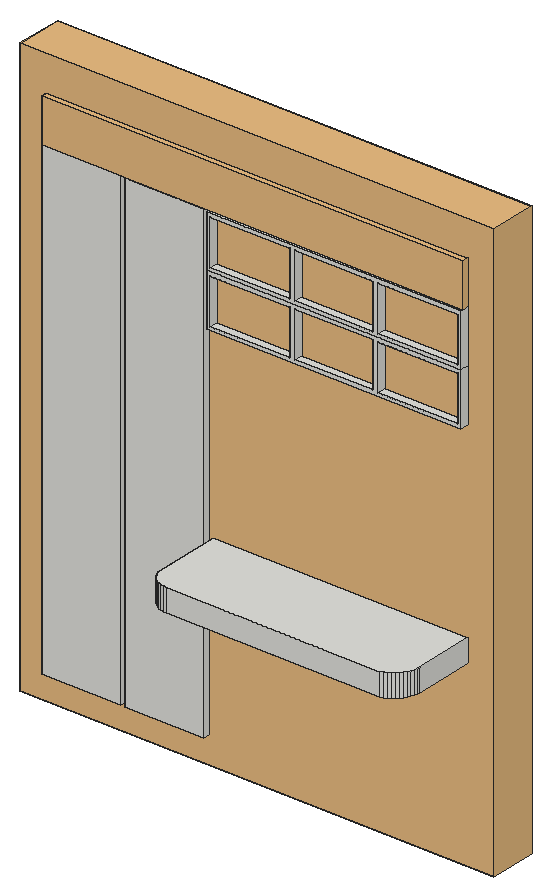
# SketchUp Ruby script. Lengths in inches.
U = 1.inch
M = Sketchup.active_model
def pt(a) = Geom::Point3d.new(a.map { |v| v * U })
def face(e, loops, mat)
  f = e.add_face(loops[0].map { |a| pt(a) })
  loops[1..].each { |l| e.add_face(l.map { |a| pt(a) }).erase! }
  f.material = f.back_material = mat if mat
  f
end
# faces: each face lists its corners as indices into pts; further lists are holes
def faces(e, pts, list, mat = nil) = list.each { |f| face(e, (f[0].is_a?(Array) ? f : [f]).map { |l| l.map { |i| pts[i] } }, mat) }
# xy, xz, yz: faces in a plane at the given z, y or x. An outline is a flat list of corners, or four numbers for a rectangle; further outlines are holes
def ring(l) = l.size == 4 ? [[l[0], l[1]], [l[2], l[1]], [l[2], l[3]], [l[0], l[3]]] : l.each_slice(2).to_a
def flat(e, list, mat, &to3) = list.each { |f| face(e, (f[0].is_a?(Array) ? f : [f]).map { |l| ring(l).map { |u, v| to3.(u, v) } }, mat) }
def xy(e, z, list, mat = nil) = flat(e, list, mat) { |x, y| [x, y, z] }
def xz(e, y, list, mat = nil) = flat(e, list, mat) { |x, z| [x, y, z] }
def yz(e, x, list, mat = nil) = flat(e, list, mat) { |y, z| [x, y, z] }
def lines(e, pts, list) = list.each { |a, b| e.add_line(pt(pts[a]), pt(pts[b])) }
# prism: a flat outline (further loops are holes) pulled along v
def prism(e, loops, v, mat = nil)
  f = face(e, loops, mat); d = Geom::Vector3d.new(v.map { |x| x * U })
  f.pushpull(f.normal.samedirection?(d) ? d.length : -d.length)
end
def box(e, o, s, mat = nil) = prism(e, [[o, [o[0] + s[0], o[1], o[2]], [o[0] + s[0], o[1] + s[1], o[2]], [o[0], o[1] + s[1], o[2]]]], [0, 0, s[2]], mat)
def at(x, y, z, deg = 0) = Geom::Transformation.translation(pt([x, y, z])) * Geom::Transformation.rotation(ORIGIN, Z_AXIS, deg.degrees)
def axes(o, x, y, z) = Geom::Transformation.new([*x, 0, *y, 0, *z, 0, *pt(o).to_a, 1])
def part(name) = M.definitions.add(name)
# library, detail: a bought-in or finely detailed component or shape, given as its bounding box
def library(name, o, s) = part(name).tap { |d| box(d.entities, o, s) }
def detail(e, o, s) = box(e.add_group.entities, o, s)
def put(e, d, t, mat = nil) = e.add_instance(d, t).tap { |i| i.material = mat if mat }
def group(e, t, mat = nil) = e.add_group.tap { |g| g.transformation = t; g.material = mat if mat }.entities
root = M.entities
c1 = library("Group\#5",[0,-12,0],[96,12,10])
xz(root,30,[[44.8,84.8,63,95.2],[64.2,84.8,81.8,95.2],[83,84.8,101.2,95.2]])
detail(root,[0,19.34,-6],[108,10.66,132])
g1 = group(root,at(0,30,-6))
xz(g1,0,[[[0,0,108,132],[5,5,103,127]]])
g2 = group(root,at(44,30,35.4))
xy(g2,0,[[4.82,-30,4.13,-29.95,3.45,-29.8,2.79,-29.56,2.18,-29.22,1.62,-28.8,1.13,-28.31,0.71,-27.75,0.38,-27.13,0.14,-26.48,0,-25.83,0,1.0625,58,1.0625,58,-24.4375,57.96,-24.89,57.82,-25.59,57.6,-26.27,57.3,-26.93,56.92,-27.54,56.48,-28.11,55.98,-28.62,55.42,-29.07,54.81,-29.46,54.16,-29.77,53.48,-30]])
xy(g2,5.2,[[4.82,-30,53.48,-30,54.16,-29.77,54.81,-29.46,55.42,-29.07,55.98,-28.62,56.48,-28.11,56.92,-27.54,57.3,-26.93,57.6,-26.27,57.82,-25.59,57.96,-24.89,58,-24.4375,58,1.0625,0,1.0625,0,-25.83,0.14,-26.48,0.38,-27.13,0.71,-27.75,1.13,-28.31,1.62,-28.8,2.18,-29.22,2.79,-29.56,3.45,-29.8,4.13,-29.95],[58,-24.4375,58.02,-24.17,58,-23.45]])
xz(g2,-30,[[4.82,0,53.48,5.2]])
xz(g2,1.0625,[[0,0,58,5.2]])
yz(g2,0,[[-25.83,0,1.0625,5.2]])
yz(g2,58,[[-24.4375,0,1.0625,5.2]])
p = [[4.13,-29.95,5.2],[3.45,-29.8,5.2],[3.45,-29.8,0],[4.13,-29.95,0],[4.82,-30,5.2],[4.82,-30,0],
  [54.16,-29.77,5.2],[53.48,-30,5.2],[53.48,-30,0],[54.16,-29.77,0],[2.79,-29.56,5.2],[2.79,-29.56,0],
  [54.81,-29.46,5.2],[54.81,-29.46,0],[2.18,-29.22,5.2],[2.18,-29.22,0],[55.42,-29.07,5.2],[55.42,-29.07,0],
  [1.62,-28.8,5.2],[1.62,-28.8,0],[55.98,-28.62,5.2],[55.98,-28.62,0],[1.13,-28.31,5.2],[1.13,-28.31,0],
  [56.48,-28.11,5.2],[56.48,-28.11,0],[0.71,-27.75,5.2],[0.71,-27.75,0],[56.92,-27.54,5.2],[56.92,-27.54,0],
  [0.38,-27.13,5.2],[0.38,-27.13,0],[57.3,-26.93,5.2],[57.3,-26.93,0],[0.14,-26.48,5.2],[0.14,-26.48,0],
  [57.6,-26.27,5.2],[57.6,-26.27,0],[0,-25.83,5.2],[0,-25.83,0],[57.82,-25.59,5.2],[57.82,-25.59,0],
  [57.96,-24.89,5.2],[57.96,-24.89,0],[58,-24.4375,5.2],[58,-24.4375,0]]
faces(g2,p,[[0,1,2,3],[4,0,3,5],[6,7,8,9],[1,10,11,2],[12,6,9,13],[10,14,15,11],[16,12,13,17],[14,18,19,15],
  [20,16,17,21],[18,22,23,19],[24,20,21,25],[22,26,27,23],[28,24,25,29],[26,30,31,27],[32,28,29,33],[30,34,35,31],
  [36,32,33,37],[34,38,39,35],[40,36,37,41],[42,40,41,43],[44,42,43,45]])
g3 = group(root,at(6,30,0))
box(g3,[0,-12,0],[18,12,108])
g4 = group(root,at(25,30,0))
box(g4,[0,-12,0],[18,12,108])
put(root,c1,at(6,30,108))
g5 = group(root,at(44,30,96))
xy(g5,0,[[0,-12.6,58,0]])
xy(g5,0.8,[[0.8,-12.6,19,0],[20.2,-12.6,37.8,0],[39,-12.6,57.2,0]])
xy(g5,11.2,[[0.8,-12.6,19,0],[20.2,-12.6,37.8,0],[39,-12.6,57.2,0]])
xy(g5,12,[[0,-12.6,58,0]])
xz(g5,-12.6,[[[0,0,58,12],[39,0.8,57.2,11.2],[0.8,0.8,19,11.2],[20.2,0.8,37.8,11.2]]])
xz(g5,0,[[[0,0,58,12],[39,0.8,57.2,11.2],[0.8,0.8,19,11.2],[20.2,0.8,37.8,11.2]],[0.8,0.8,19,11.2],[20.2,0.8,37.8,11.2],[39,0.8,57.2,11.2]])
yz(g5,0,[[-12.6,0,0,12]])
yz(g5,0.8,[[-12.6,0.8,0,11.2]])
yz(g5,19,[[-12.6,0.8,0,11.2]])
yz(g5,20.2,[[-12.6,0.8,0,11.2]])
yz(g5,37.8,[[-12.6,0.8,0,11.2]])
yz(g5,39,[[-12.6,0.8,0,11.2]])
yz(g5,57.2,[[-12.6,0.8,0,11.2]])
yz(g5,58,[[-12.6,0,0,12]])
g6 = group(root,at(44,30,84))
prism(g6,[[[0,0,0],[0,0,12],[58,0,12],[58,0,0]],[[39,0,0.8],[57.2,0,0.8],[57.2,0,11.2],[39,0,11.2]],[[19,0,0.8],[19,0,11.2],[0.8,0,11.2],[0.8,0,0.8]],[[37.8,0,0.8],[37.8,0,11.2],[20.2,0,11.2],[20.2,0,0.8]]],[0,-12.6,0])
